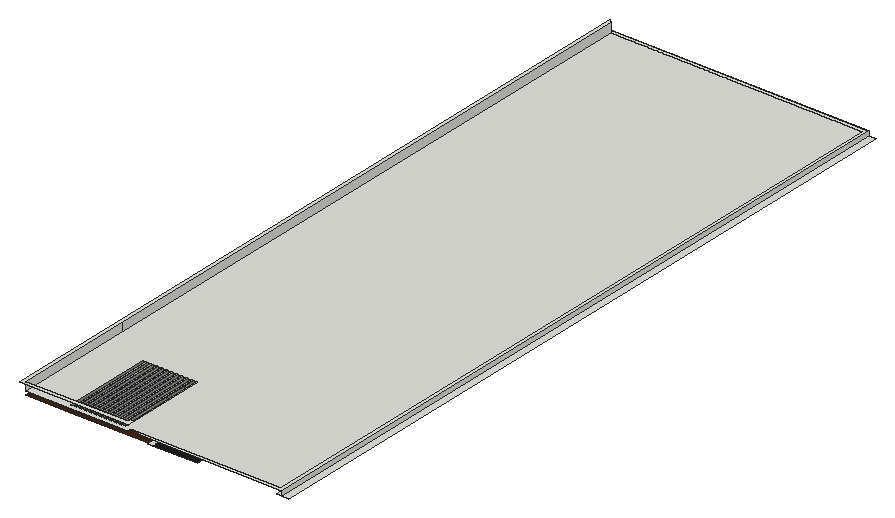
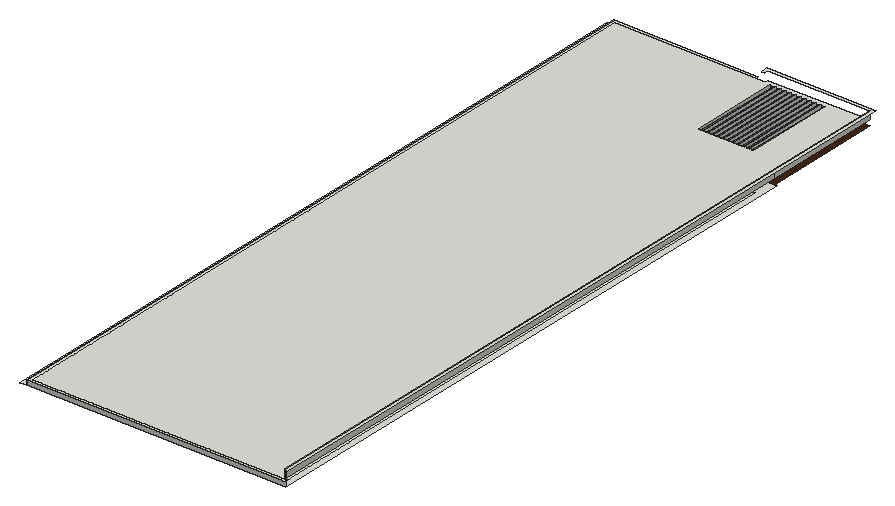
# SketchUp Ruby script. Lengths in inches.
U = 1.inch
M = Sketchup.active_model
def pt(a) = Geom::Point3d.new(a.map { |v| v * U })
def face(e, loops, mat)
  f = e.add_face(loops[0].map { |a| pt(a) })
  loops[1..].each { |l| e.add_face(l.map { |a| pt(a) }).erase! }
  f.material = f.back_material = mat if mat
  f
end
# faces: each face lists its corners as indices into pts; further lists are holes
def faces(e, pts, list, mat = nil) = list.each { |f| face(e, (f[0].is_a?(Array) ? f : [f]).map { |l| l.map { |i| pts[i] } }, mat) }
# xy, xz, yz: faces in a plane at the given z, y or x. An outline is a flat list of corners, or four numbers for a rectangle; further outlines are holes
def ring(l) = l.size == 4 ? [[l[0], l[1]], [l[2], l[1]], [l[2], l[3]], [l[0], l[3]]] : l.each_slice(2).to_a
def flat(e, list, mat, &to3) = list.each { |f| face(e, (f[0].is_a?(Array) ? f : [f]).map { |l| ring(l).map { |u, v| to3.(u, v) } }, mat) }
def xy(e, z, list, mat = nil) = flat(e, list, mat) { |x, y| [x, y, z] }
def xz(e, y, list, mat = nil) = flat(e, list, mat) { |x, z| [x, y, z] }
def yz(e, x, list, mat = nil) = flat(e, list, mat) { |y, z| [x, y, z] }
def lines(e, pts, list) = list.each { |a, b| e.add_line(pt(pts[a]), pt(pts[b])) }
# prism: a flat outline (further loops are holes) pulled along v
def prism(e, loops, v, mat = nil)
  f = face(e, loops, mat); d = Geom::Vector3d.new(v.map { |x| x * U })
  f.pushpull(f.normal.samedirection?(d) ? d.length : -d.length)
end
def box(e, o, s, mat = nil) = prism(e, [[o, [o[0] + s[0], o[1], o[2]], [o[0] + s[0], o[1] + s[1], o[2]], [o[0], o[1] + s[1], o[2]]]], [0, 0, s[2]], mat)
def at(x, y, z, deg = 0) = Geom::Transformation.translation(pt([x, y, z])) * Geom::Transformation.rotation(ORIGIN, Z_AXIS, deg.degrees)
def axes(o, x, y, z) = Geom::Transformation.new([*x, 0, *y, 0, *z, 0, *pt(o).to_a, 1])
def part(name) = M.definitions.add(name)
# library, detail: a bought-in or finely detailed component or shape, given as its bounding box
def library(name, o, s) = part(name).tap { |d| box(d.entities, o, s) }
def detail(e, o, s) = box(e.add_group.entities, o, s)
def put(e, d, t, mat = nil) = e.add_instance(d, t).tap { |i| i.material = mat if mat }
def group(e, t, mat = nil) = e.add_group.tap { |g| g.transformation = t; g.material = mat if mat }.entities
root = M.entities
M.materials.add("[Color M08]").color = [30, 30, 30]
M.materials.add("[Field Square Tile]").color = [211, 167, 108]
M.materials.add("[Granite Light Gray]").color = [149, 148, 144]
M.materials.add("[Wood Veneer 01]").color = [66, 38, 20]
xy(root,380.5,[[3312.79,2346.71,3312.79,3661.44,2865.03,3661.44,2865.03,2597.8,3081.03,2597.8,3081.03,2562.82,2855.22,2562.82,2855.22,3671.25,3322.6,3671.25,3322.6,2346.71],[3081.03,2346.71,3089.95,2425.46],[3322.6,2346.71,3334.41,3671.25],[3081.03,2425.46,3081.03,2597.8,2865.03,2597.8,2865.03,3661.44,3312.79,3661.44,3312.79,2425.46,3266.02,2425.46,3266.02,2532.83,3170.71,2532.83,3170.71,2573.65,3089.95,2573.65,3089.95,2532.83,3081.33,2532.83,3081.33,2425.46],[3081.33,2425.46,3089.95,2532.83],
  [3170.71,2425.46,3266.02,2532.83],[3089.95,2532.83,3170.71,2573.65]])
xy(root,380.5,[[3089.95,2346.71,3170.71,2532.83]],"[Color M08]")
xy(root,380.5,[[[2860.05,2347.9,2931.98,2562.82],[2916.83,2501.63,2918.35,2502.01,2919.73,2502.76,2920.86,2503.84,2921.67,2505.18,2922.1,2506.6875,2922.14,2508.25,2921.76,2509.78,2921.01,2511.15,2919.92,2512.28,2918.58,2513.09,2917.08,2513.53,2915.51,2513.56,2913.99,2513.19,2912.62,2512.43,2911.49,2511.35,2910.68,2510.01,2910.24,2508.5,2910.21,2506.9375,2910.58,2505.41,2911.34,2504.04,2912.42,2502.91,2913.76,2502.1,2915.27,2501.66],[2916.83,2441.63,2918.35,2442.01,2919.73,2442.76,2920.86,2443.84,2921.67,2445.18,2922.1,2446.6875,2922.14,2448.25,2921.76,2449.78,2921.01,2451.15,2919.92,2452.28,2918.58,2453.09,2917.08,2453.53,2915.51,2453.56,2913.99,2453.19,2912.62,2452.43,2911.49,2451.35,2910.68,2450.01,2910.24,2448.5,2910.21,2446.9375,2910.58,2445.41,2911.34,2444.04,2912.42,2442.91,2913.76,2442.1,2915.27,2441.66],[2916.83,2389.88,2918.35,2390.26,2919.73,2391.01,2920.86,2392.09,2921.67,2393.43,2922.1,2394.9375,2922.14,2396.5,2921.76,2398.03,2921.01,2399.4,2919.92,2400.53,2918.58,2401.34,2917.08,2401.78,2915.51,2401.81,2913.99,2401.44,2912.62,2400.68,2911.49,2399.6,2910.68,2398.26,2910.24,2396.75,2910.21,2395.1875,2910.58,2393.66,2911.34,2392.29,2912.42,2391.16,2913.76,2390.35,2915.27,2389.91],[2916.83,2359.13,2918.35,2359.51,2919.73,2360.26,2920.86,2361.34,2921.67,2362.68,2922.1,2364.1875,2922.14,2365.75,2921.76,2367.28,2921.01,2368.65,2919.92,2369.78,2918.58,2370.59,2917.08,2371.03,2915.51,2371.06,2913.99,2370.69,2912.62,2369.93,2911.49,2368.85,2910.68,2367.51,2910.24,2366,2910.21,2364.4375,2910.58,2362.91,2911.34,2361.54,2912.42,2360.41,2913.76,2359.6,2915.27,2359.16],[2877.08,2441.63,2878.6,2442.01,2879.98,2442.76,2881.11,2443.84,2881.92,2445.18,2882.35,2446.6875,2882.39,2448.25,2882.01,2449.78,2881.26,2451.15,2880.17,2452.28,2878.83,2453.09,2877.33,2453.53,2875.76,2453.56,2874.24,2453.19,2872.87,2452.43,2871.74,2451.35,2870.93,2450.01,2870.49,2448.5,2870.46,2446.9375,2870.83,2445.41,2871.59,2444.04,2872.67,2442.91,2874.01,2442.1,2875.52,2441.66],[2877.08,2389.88,2878.6,2390.26,2879.98,2391.01,2881.11,2392.09,2881.92,2393.43,2882.35,2394.9375,2882.39,2396.5,2882.01,2398.03,2881.26,2399.4,2880.17,2400.53,2878.83,2401.34,2877.33,2401.78,2875.76,2401.81,2874.24,2401.44,2872.87,2400.68,2871.74,2399.6,2870.93,2398.26,2870.49,2396.75,2870.46,2395.1875,2870.83,2393.66,2871.59,2392.29,2872.67,2391.16,2874.01,2390.35,2875.52,2389.91],[2877.08,2359.13,2878.6,2359.51,2879.98,2360.26,2881.11,2361.34,2881.92,2362.68,2882.35,2364.1875,2882.39,2365.75,2882.01,2367.28,2881.26,2368.65,2880.17,2369.78,2878.83,2370.59,2877.33,2371.03,2875.76,2371.06,2874.24,2370.69,2872.87,2369.93,2871.74,2368.85,2870.93,2367.51,2870.49,2366,2870.46,2364.4375,2870.83,2362.91,2871.59,2361.54,2872.67,2360.41,2874.01,2359.6,2875.52,2359.16],[2877.08,2501.63,2878.6,2502.01,2879.98,2502.76,2881.11,2503.84,2881.92,2505.18,2882.35,2506.6875,2882.39,2508.25,2882.01,2509.78,2881.26,2511.15,2880.17,2512.28,2878.83,2513.09,2877.33,2513.53,2875.76,2513.56,2874.24,2513.19,2872.87,2512.43,2871.74,2511.35,2870.93,2510.01,2870.49,2508.5,2870.46,2506.9375,2870.83,2505.41,2871.59,2504.04,2872.67,2502.91,2874.01,2502.1,2875.52,2501.66]],[[2931.98,2347.9,3081.03,2562.82],[3027.43,2355.06,3033.68,2516.12],[3018.31,2355.06,3024.56,2516.12],[3009.18,2355.06,3015.43,2516.12],[3000.06,2355.06,3006.31,2516.12],[2990.93,2355.06,2997.18,2516.12],[2981.81,2355.06,2988.06,2516.12],[2972.68,2355.06,2978.93,2516.12],[2963.56,2355.06,2969.81,2516.12],[2954.43,2355.06,2960.68,2516.12],[2945.31,2355.06,2951.56,2516.12],[2936.18,2355.06,2942.43,2516.12]]],"[Wood Veneer 01]")
xy(root,381.875,[[2877.08,2389.88,2875.52,2389.91,2874.01,2390.35,2872.67,2391.16,2871.59,2392.29,2870.83,2393.66,2870.46,2395.1875,2870.49,2396.75,2870.93,2398.26,2871.74,2399.6,2872.87,2400.68,2874.24,2401.44,2875.76,2401.81,2877.33,2401.78,2878.83,2401.34,2880.17,2400.53,2881.26,2399.4,2882.01,2398.03,2882.39,2396.5,2882.35,2394.9375,2881.92,2393.43,2881.11,2392.09,2879.98,2391.01,2878.6,2390.26],[2916.83,2389.88,2915.27,2389.91,2913.76,2390.35,2912.42,2391.16,2911.34,2392.29,2910.58,2393.66,2910.21,2395.1875,2910.24,2396.75,2910.68,2398.26,2911.49,2399.6,2912.62,2400.68,2913.99,2401.44,2915.51,2401.81,2917.08,2401.78,2918.58,2401.34,2919.92,2400.53,2921.01,2399.4,2921.76,2398.03,2922.14,2396.5,2922.1,2394.9375,2921.67,2393.43,2920.86,2392.09,2919.73,2391.01,2918.35,2390.26],[2877.08,2441.63,2875.52,2441.66,2874.01,2442.1,2872.67,2442.91,2871.59,2444.04,2870.83,2445.41,2870.46,2446.9375,2870.49,2448.5,2870.93,2450.01,2871.74,2451.35,2872.87,2452.43,2874.24,2453.19,2875.76,2453.56,2877.33,2453.53,2878.83,2453.09,2880.17,2452.28,2881.26,2451.15,2882.01,2449.78,2882.39,2448.25,2882.35,2446.6875,2881.92,2445.18,2881.11,2443.84,2879.98,2442.76,2878.6,2442.01],[2916.83,2441.63,2915.27,2441.66,2913.76,2442.1,2912.42,2442.91,2911.34,2444.04,2910.58,2445.41,2910.21,2446.9375,2910.24,2448.5,2910.68,2450.01,2911.49,2451.35,2912.62,2452.43,2913.99,2453.19,2915.51,2453.56,2917.08,2453.53,2918.58,2453.09,2919.92,2452.28,2921.01,2451.15,2921.76,2449.78,2922.14,2448.25,2922.1,2446.6875,2921.67,2445.18,2920.86,2443.84,2919.73,2442.76,2918.35,2442.01],[2877.08,2501.63,2875.52,2501.66,2874.01,2502.1,2872.67,2502.91,2871.59,2504.04,2870.83,2505.41,2870.46,2506.9375,2870.49,2508.5,2870.93,2510.01,2871.74,2511.35,2872.87,2512.43,2874.24,2513.19,2875.76,2513.56,2877.33,2513.53,2878.83,2513.09,2880.17,2512.28,2881.26,2511.15,2882.01,2509.78,2882.39,2508.25,2882.35,2506.6875,2881.92,2505.18,2881.11,2503.84,2879.98,2502.76,2878.6,2502.01],
  [2916.83,2501.63,2915.27,2501.66,2913.76,2502.1,2912.42,2502.91,2911.34,2504.04,2910.58,2505.41,2910.21,2506.9375,2910.24,2508.5,2910.68,2510.01,2911.49,2511.35,2912.62,2512.43,2913.99,2513.19,2915.51,2513.56,2917.08,2513.53,2918.58,2513.09,2919.92,2512.28,2921.01,2511.15,2921.76,2509.78,2922.14,2508.25,2922.1,2506.6875,2921.67,2505.18,2920.86,2503.84,2919.73,2502.76,2918.35,2502.01]],"[Field Square Tile]")
xy(root,388.625,[[[2861.56,2346.49,3044.88,2346.49,3044.88,2353.05,3316.25,2353.05,3316.25,3664.91,2861.56,3664.91],[2936.18,2355.06,2942.43,2516.12],[2945.31,2355.06,2951.56,2516.12],[2954.43,2355.06,2960.68,2516.12],[2963.56,2355.06,2969.81,2516.12],[2972.68,2355.06,2978.93,2516.12],[2981.81,2355.06,2988.06,2516.12],[2990.93,2355.06,2997.18,2516.12],[3000.06,2355.06,3006.31,2516.12],[3009.18,2355.06,3015.43,2516.12],[3018.31,2355.06,3024.56,2516.12],[3027.43,2355.06,3033.68,2516.12]],[3061.9375,2346.71,3322.6,2346.71,3322.6,3671.25,2855.22,3671.25,2861.56,3664.91,3316.25,3664.91,3316.25,2353.05,3061.9375,2353.05]])
xy(root,403.8125,[[2855.22,2340.15,3051.23,2340.15,3051.23,2353.05,3044.88,2353.05,3044.88,2346.49,2861.56,2346.49,2861.56,3664.91,2855.22,3671.25]])
xz(root,2516.12,[[2936.18,380.5,2942.43,388.625],[2945.31,380.5,2951.56,388.625],[2954.43,380.5,2960.68,388.625],[2963.56,380.5,2969.81,388.625],[2972.68,380.5,2978.93,388.625],
  [2981.81,380.5,2988.06,388.625],[2990.93,380.5,2997.18,388.625],[3000.06,380.5,3006.31,388.625],[3009.18,380.5,3015.43,388.625],[3018.31,380.5,3024.56,388.625],
  [3027.43,380.5,3033.68,388.625]],"[Granite Light Gray]")
xz(root,3671.25,[[2855.22,380.5,3322.6,388.625]])
yz(root,2861.56,[[2346.49,388.625,2562.82,403.8125],[2562.82,388.625,3664.91,403.8125]])
yz(root,2936.18,[[2355.06,380.5,2516.12,388.625]],"[Granite Light Gray]")
yz(root,2942.43,[[2355.06,380.5,2516.12,388.625]])
yz(root,2945.31,[[2355.06,380.5,2516.12,388.625]],"[Granite Light Gray]")
yz(root,2951.56,[[2355.06,380.5,2516.12,388.625]])
yz(root,2954.43,[[2355.06,380.5,2516.12,388.625]],"[Granite Light Gray]")
yz(root,2960.68,[[2355.06,380.5,2516.12,388.625]])
yz(root,2963.56,[[2355.06,380.5,2516.12,388.625]],"[Granite Light Gray]")
yz(root,2969.81,[[2355.06,380.5,2516.12,388.625]])
yz(root,2972.68,[[2355.06,380.5,2516.12,388.625]],"[Granite Light Gray]")
yz(root,2978.93,[[2355.06,380.5,2516.12,388.625]])
yz(root,2981.81,[[2355.06,380.5,2516.12,388.625]],"[Granite Light Gray]")
yz(root,2988.06,[[2355.06,380.5,2516.12,388.625]])
yz(root,2990.93,[[2355.06,380.5,2516.12,388.625]],"[Granite Light Gray]")
yz(root,2997.18,[[2355.06,380.5,2516.12,388.625]])
yz(root,3000.06,[[2355.06,380.5,2516.12,388.625]],"[Granite Light Gray]")
yz(root,3006.31,[[2355.06,380.5,2516.12,388.625]])
yz(root,3009.18,[[2355.06,380.5,2516.12,388.625]],"[Granite Light Gray]")
yz(root,3015.43,[[2355.06,380.5,2516.12,388.625]])
yz(root,3018.31,[[2355.06,380.5,2516.12,388.625]],"[Granite Light Gray]")
yz(root,3024.56,[[2355.06,380.5,2516.12,388.625]])
yz(root,3027.43,[[2355.06,380.5,2516.12,388.625]],"[Granite Light Gray]")
yz(root,3033.68,[[2355.06,380.5,2516.12,388.625]])
yz(root,3322.6,[[2346.71,380.5,3671.25,388.625]])
p = [[2875.76,2371.06,380.5],[2877.33,2371.03,380.5],[2877.33,2371.03,381.875],[2875.76,2371.06,381.875],[2915.51,2371.06,380.5],[2917.08,2371.03,380.5],
  [2917.08,2371.03,381.875],[2915.51,2371.06,381.875],[2875.52,2389.91,380.5],[2874.01,2390.35,380.5],[2874.01,2390.35,381.875],[2875.52,2389.91,381.875],
  [2877.08,2389.88,380.5],[2877.08,2389.88,381.875],[2878.6,2390.26,380.5],[2878.6,2390.26,381.875],[2915.27,2389.91,380.5],[2913.76,2390.35,380.5],
  [2913.76,2390.35,381.875],[2915.27,2389.91,381.875],[2916.83,2389.88,380.5],[2916.83,2389.88,381.875],[2918.35,2390.26,380.5],[2918.35,2390.26,381.875],
  [2879.98,2391.01,380.5],[2879.98,2391.01,381.875],[2919.73,2391.01,380.5],[2919.73,2391.01,381.875],[2872.67,2391.16,380.5],[2872.67,2391.16,381.875],
  [2912.42,2391.16,380.5],[2912.42,2391.16,381.875],[2881.11,2392.09,380.5],[2881.11,2392.09,381.875],[2920.86,2392.09,380.5],[2920.86,2392.09,381.875],
  [2871.59,2392.29,380.5],[2871.59,2392.29,381.875],[2911.34,2392.29,380.5],[2911.34,2392.29,381.875],[2881.92,2393.43,380.5],[2881.92,2393.43,381.875],
  [2921.67,2393.43,380.5],[2921.67,2393.43,381.875],[2870.83,2393.66,380.5],[2870.83,2393.66,381.875],[2910.58,2393.66,380.5],[2910.58,2393.66,381.875],
  [2882.35,2394.9375,380.5],[2882.35,2394.9375,381.875],[2922.1,2394.9375,380.5],[2922.1,2394.9375,381.875],[2870.46,2395.1875,380.5],[2870.46,2395.1875,381.875],
  [2910.21,2395.1875,380.5],[2910.21,2395.1875,381.875],[2882.39,2396.5,380.5],[2882.39,2396.5,381.875],[2922.14,2396.5,380.5],[2922.14,2396.5,381.875],
  [2870.49,2396.75,380.5],[2870.49,2396.75,381.875],[2910.24,2396.75,380.5],[2910.24,2396.75,381.875],[2882.01,2398.03,380.5],[2882.01,2398.03,381.875],
  [2921.76,2398.03,380.5],[2921.76,2398.03,381.875],[2870.93,2398.26,380.5],[2870.93,2398.26,381.875],[2910.68,2398.26,380.5],[2910.68,2398.26,381.875],
  [2881.26,2399.4,380.5],[2881.26,2399.4,381.875],[2921.01,2399.4,380.5],[2921.01,2399.4,381.875],[2871.74,2399.6,380.5],[2871.74,2399.6,381.875],
  [2911.49,2399.6,380.5],[2911.49,2399.6,381.875],[2880.17,2400.53,380.5],[2880.17,2400.53,381.875],[2919.92,2400.53,380.5],[2919.92,2400.53,381.875],
  [2872.87,2400.68,380.5],[2872.87,2400.68,381.875],[2912.62,2400.68,380.5],[2912.62,2400.68,381.875],[2878.83,2401.34,380.5],[2878.83,2401.34,381.875],
  [2918.58,2401.34,380.5],[2918.58,2401.34,381.875],[2874.24,2401.44,380.5],[2874.24,2401.44,381.875],[2913.99,2401.44,380.5],[2913.99,2401.44,381.875],
  [2877.33,2401.78,380.5],[2877.33,2401.78,381.875],[2917.08,2401.78,380.5],[2917.08,2401.78,381.875],[2875.76,2401.81,380.5],[2875.76,2401.81,381.875],
  [2915.51,2401.81,380.5],[2915.51,2401.81,381.875],[2877.08,2441.63,380.5],[2875.52,2441.66,380.5],[2875.52,2441.66,381.875],[2877.08,2441.63,381.875],
  [2878.6,2442.01,380.5],[2878.6,2442.01,381.875],[2916.83,2441.63,380.5],[2915.27,2441.66,380.5],[2915.27,2441.66,381.875],[2916.83,2441.63,381.875],
  [2918.35,2442.01,380.5],[2918.35,2442.01,381.875],[2874.01,2442.1,380.5],[2874.01,2442.1,381.875],[2913.76,2442.1,380.5],[2913.76,2442.1,381.875],
  [2879.98,2442.76,380.5],[2879.98,2442.76,381.875],[2919.73,2442.76,380.5],[2919.73,2442.76,381.875],[2872.67,2442.91,380.5],[2872.67,2442.91,381.875],
  [2912.42,2442.91,380.5],[2912.42,2442.91,381.875],[2881.11,2443.84,380.5],[2881.11,2443.84,381.875],[2920.86,2443.84,380.5],[2920.86,2443.84,381.875],
  [2871.59,2444.04,380.5],[2871.59,2444.04,381.875],[2911.34,2444.04,380.5],[2911.34,2444.04,381.875],[2881.92,2445.18,380.5],[2881.92,2445.18,381.875],
  [2921.67,2445.18,380.5],[2921.67,2445.18,381.875],[2870.83,2445.41,380.5],[2870.83,2445.41,381.875],[2910.58,2445.41,380.5],[2910.58,2445.41,381.875],
  [2882.35,2446.6875,380.5],[2882.35,2446.6875,381.875],[2922.1,2446.6875,380.5],[2922.1,2446.6875,381.875],[2870.46,2446.9375,380.5],[2870.46,2446.9375,381.875],
  [2910.21,2446.9375,380.5],[2910.21,2446.9375,381.875],[2882.39,2448.25,380.5],[2882.39,2448.25,381.875],[2922.14,2448.25,380.5],[2922.14,2448.25,381.875],
  [2870.49,2448.5,380.5],[2870.49,2448.5,381.875],[2910.24,2448.5,380.5],[2910.24,2448.5,381.875],[2882.01,2449.78,380.5],[2882.01,2449.78,381.875],
  [2921.76,2449.78,380.5],[2921.76,2449.78,381.875],[2870.93,2450.01,380.5],[2870.93,2450.01,381.875],[2910.68,2450.01,380.5],[2910.68,2450.01,381.875],
  [2881.26,2451.15,380.5],[2881.26,2451.15,381.875],[2921.01,2451.15,380.5],[2921.01,2451.15,381.875],[2871.74,2451.35,380.5],[2871.74,2451.35,381.875],
  [2911.49,2451.35,380.5],[2911.49,2451.35,381.875],[2880.17,2452.28,380.5],[2880.17,2452.28,381.875],[2919.92,2452.28,380.5],[2919.92,2452.28,381.875],
  [2872.87,2452.43,380.5],[2872.87,2452.43,381.875],[2912.62,2452.43,380.5],[2912.62,2452.43,381.875],[2878.83,2453.09,380.5],[2878.83,2453.09,381.875],
  [2918.58,2453.09,380.5],[2918.58,2453.09,381.875],[2874.24,2453.19,380.5],[2874.24,2453.19,381.875],[2913.99,2453.19,380.5],[2913.99,2453.19,381.875],
  [2877.33,2453.53,380.5],[2877.33,2453.53,381.875],[2917.08,2453.53,380.5],[2917.08,2453.53,381.875],[2875.76,2453.56,380.5],[2875.76,2453.56,381.875],
  [2915.51,2453.56,380.5],[2915.51,2453.56,381.875],[2877.08,2501.63,380.5],[2875.52,2501.66,380.5],[2875.52,2501.66,381.875],[2877.08,2501.63,381.875],
  [2878.6,2502.01,380.5],[2878.6,2502.01,381.875],[2916.83,2501.63,380.5],[2915.27,2501.66,380.5],[2915.27,2501.66,381.875],[2916.83,2501.63,381.875],
  [2918.35,2502.01,380.5],[2918.35,2502.01,381.875],[2874.01,2502.1,380.5],[2874.01,2502.1,381.875],[2913.76,2502.1,380.5],[2913.76,2502.1,381.875],
  [2879.98,2502.76,380.5],[2879.98,2502.76,381.875],[2919.73,2502.76,380.5],[2919.73,2502.76,381.875],[2872.67,2502.91,380.5],[2872.67,2502.91,381.875],
  [2912.42,2502.91,380.5],[2912.42,2502.91,381.875],[2881.11,2503.84,380.5],[2881.11,2503.84,381.875],[2920.86,2503.84,380.5],[2920.86,2503.84,381.875],
  [2871.59,2504.04,380.5],[2871.59,2504.04,381.875],[2911.34,2504.04,380.5],[2911.34,2504.04,381.875],[2881.92,2505.18,380.5],[2881.92,2505.18,381.875],
  [2921.67,2505.18,380.5],[2921.67,2505.18,381.875],[2870.83,2505.41,380.5],[2870.83,2505.41,381.875],[2910.58,2505.41,380.5],[2910.58,2505.41,381.875],
  [2882.35,2506.6875,380.5],[2882.35,2506.6875,381.875],[2922.1,2506.6875,380.5],[2922.1,2506.6875,381.875],[2870.46,2506.9375,380.5],[2870.46,2506.9375,381.875],
  [2910.21,2506.9375,380.5],[2910.21,2506.9375,381.875],[2882.39,2508.25,380.5],[2882.39,2508.25,381.875],[2922.14,2508.25,380.5],[2922.14,2508.25,381.875],
  [2870.49,2508.5,380.5],[2870.49,2508.5,381.875],[2910.24,2508.5,380.5],[2910.24,2508.5,381.875],[2882.01,2509.78,380.5],[2882.01,2509.78,381.875],
  [2921.76,2509.78,380.5],[2921.76,2509.78,381.875],[2870.93,2510.01,380.5],[2870.93,2510.01,381.875],[2910.68,2510.01,380.5],[2910.68,2510.01,381.875],
  [2881.26,2511.15,380.5],[2881.26,2511.15,381.875],[2921.01,2511.15,380.5],[2921.01,2511.15,381.875],[2871.74,2511.35,380.5],[2871.74,2511.35,381.875],
  [2911.49,2511.35,380.5],[2911.49,2511.35,381.875],[2880.17,2512.28,380.5],[2880.17,2512.28,381.875],[2919.92,2512.28,380.5],[2919.92,2512.28,381.875],
  [2872.87,2512.43,380.5],[2872.87,2512.43,381.875],[2912.62,2512.43,380.5],[2912.62,2512.43,381.875],[2878.83,2513.09,380.5],[2878.83,2513.09,381.875],
  [2918.58,2513.09,380.5],[2918.58,2513.09,381.875],[2874.24,2513.19,380.5],[2874.24,2513.19,381.875],[2913.99,2513.19,380.5],[2913.99,2513.19,381.875],
  [2877.33,2513.53,380.5],[2877.33,2513.53,381.875],[2917.08,2513.53,380.5],[2917.08,2513.53,381.875],[2875.76,2513.56,380.5],[2875.76,2513.56,381.875],
  [2915.51,2513.56,380.5],[2915.51,2513.56,381.875],[2861.56,3664.91,388.625],[2855.22,3671.25,388.625],[2855.22,3671.25,403.8125],[2861.56,3664.91,403.8125]]
faces(root,p,[[0,1,2,3],[4,5,6,7],[8,9,10,11],[12,8,11,13],[14,12,13,15],[16,17,18,19],[20,16,19,21],[22,20,21,23],
  [24,14,15,25],[26,22,23,27],[9,28,29,10],[17,30,31,18],[32,24,25,33],[34,26,27,35],[28,36,37,29],[30,38,39,31],
  [40,32,33,41],[42,34,35,43],[36,44,45,37],[38,46,47,39],[48,40,41,49],[50,42,43,51],[44,52,53,45],[46,54,55,47],
  [56,48,49,57],[58,50,51,59],[52,60,61,53],[54,62,63,55],[64,56,57,65],[66,58,59,67],[60,68,69,61],[62,70,71,63],
  [72,64,65,73],[74,66,67,75],[68,76,77,69],[70,78,79,71],[80,72,73,81],[82,74,75,83],[76,84,85,77],[78,86,87,79],
  [88,80,81,89],[90,82,83,91],[84,92,93,85],[86,94,95,87],[96,88,89,97],[98,90,91,99],[92,100,101,93],[94,102,103,95],
  [100,96,97,101],[102,98,99,103],[104,105,106,107],[108,104,107,109],[110,111,112,113],[114,110,113,115],[105,116,117,106],[111,118,119,112],
  [120,108,109,121],[122,114,115,123],[116,124,125,117],[118,126,127,119],[128,120,121,129],[130,122,123,131],[124,132,133,125],[126,134,135,127],
  [136,128,129,137],[138,130,131,139],[132,140,141,133],[134,142,143,135],[144,136,137,145],[146,138,139,147],[140,148,149,141],[142,150,151,143],
  [152,144,145,153],[154,146,147,155],[148,156,157,149],[150,158,159,151],[160,152,153,161],[162,154,155,163],[156,164,165,157],[158,166,167,159],
  [168,160,161,169],[170,162,163,171],[164,172,173,165],[166,174,175,167],[176,168,169,177],[178,170,171,179],[172,180,181,173],[174,182,183,175],
  [184,176,177,185],[186,178,179,187],[180,188,189,181],[182,190,191,183],[192,184,185,193],[194,186,187,195],[188,196,197,189],[190,198,199,191],
  [196,192,193,197],[198,194,195,199],[200,201,202,203],[204,200,203,205],[206,207,208,209],[210,206,209,211],[201,212,213,202],[207,214,215,208],
  [216,204,205,217],[218,210,211,219],[212,220,221,213],[214,222,223,215],[224,216,217,225],[226,218,219,227],[220,228,229,221],[222,230,231,223],
  [232,224,225,233],[234,226,227,235],[228,236,237,229],[230,238,239,231],[240,232,233,241],[242,234,235,243],[236,244,245,237],[238,246,247,239],
  [248,240,241,249],[250,242,243,251],[244,252,253,245],[246,254,255,247],[256,248,249,257],[258,250,251,259],[252,260,261,253],[254,262,263,255],
  [264,256,257,265],[266,258,259,267],[260,268,269,261],[262,270,271,263],[272,264,265,273],[274,266,267,275],[268,276,277,269],[270,278,279,271],
  [280,272,273,281],[282,274,275,283],[276,284,285,277],[278,286,287,279],[288,280,281,289],[290,282,283,291],[284,292,293,285],[286,294,295,287],
  [292,288,289,293],[294,290,291,295]],"[Field Square Tile]")
faces(root,p,[[296,297,298,299]])
